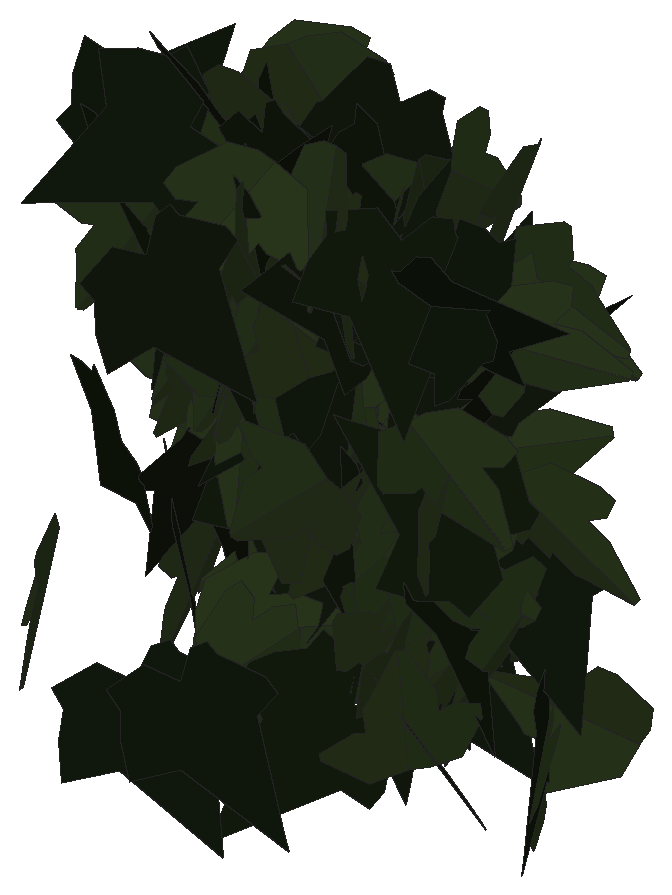
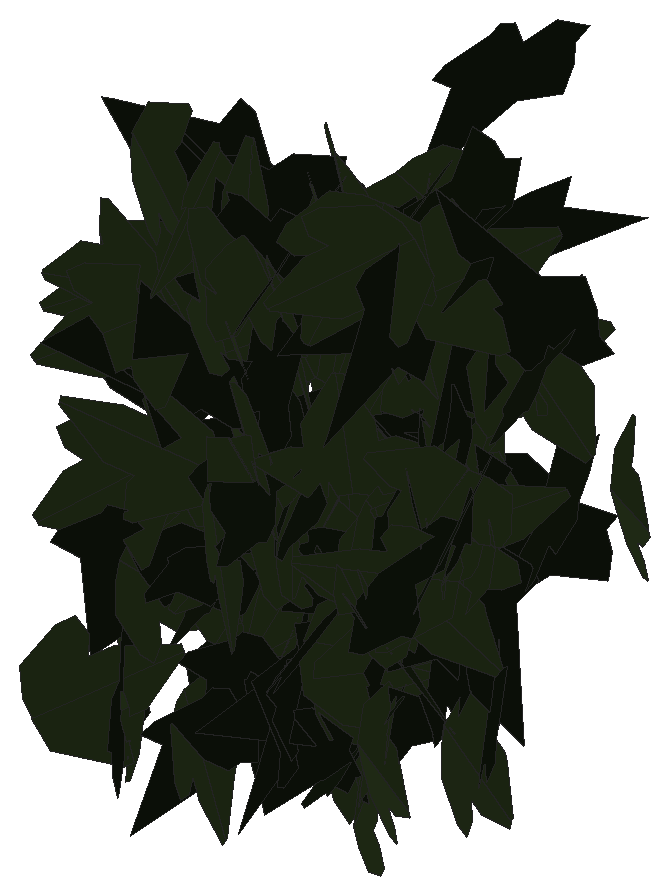
# SketchUp Ruby script. Lengths in inches.
U = 1.inch
M = Sketchup.active_model
def pt(a) = Geom::Point3d.new(a.map { |v| v * U })
def face(e, loops, mat)
  f = e.add_face(loops[0].map { |a| pt(a) })
  loops[1..].each { |l| e.add_face(l.map { |a| pt(a) }).erase! }
  f.material = f.back_material = mat if mat
  f
end
# faces: each face lists its corners as indices into pts; further lists are holes
def faces(e, pts, list, mat = nil) = list.each { |f| face(e, (f[0].is_a?(Array) ? f : [f]).map { |l| l.map { |i| pts[i] } }, mat) }
# xy, xz, yz: faces in a plane at the given z, y or x. An outline is a flat list of corners, or four numbers for a rectangle; further outlines are holes
def ring(l) = l.size == 4 ? [[l[0], l[1]], [l[2], l[1]], [l[2], l[3]], [l[0], l[3]]] : l.each_slice(2).to_a
def flat(e, list, mat, &to3) = list.each { |f| face(e, (f[0].is_a?(Array) ? f : [f]).map { |l| ring(l).map { |u, v| to3.(u, v) } }, mat) }
def xy(e, z, list, mat = nil) = flat(e, list, mat) { |x, y| [x, y, z] }
def xz(e, y, list, mat = nil) = flat(e, list, mat) { |x, z| [x, y, z] }
def yz(e, x, list, mat = nil) = flat(e, list, mat) { |y, z| [x, y, z] }
def lines(e, pts, list) = list.each { |a, b| e.add_line(pt(pts[a]), pt(pts[b])) }
# prism: a flat outline (further loops are holes) pulled along v
def prism(e, loops, v, mat = nil)
  f = face(e, loops, mat); d = Geom::Vector3d.new(v.map { |x| x * U })
  f.pushpull(f.normal.samedirection?(d) ? d.length : -d.length)
end
def box(e, o, s, mat = nil) = prism(e, [[o, [o[0] + s[0], o[1], o[2]], [o[0] + s[0], o[1] + s[1], o[2]], [o[0], o[1] + s[1], o[2]]]], [0, 0, s[2]], mat)
def at(x, y, z, deg = 0) = Geom::Transformation.translation(pt([x, y, z])) * Geom::Transformation.rotation(ORIGIN, Z_AXIS, deg.degrees)
def axes(o, x, y, z) = Geom::Transformation.new([*x, 0, *y, 0, *z, 0, *pt(o).to_a, 1])
def part(name) = M.definitions.add(name)
# library, detail: a bought-in or finely detailed component or shape, given as its bounding box
def library(name, o, s) = part(name).tap { |d| box(d.entities, o, s) }
def detail(e, o, s) = box(e.add_group.entities, o, s)
def put(e, d, t, mat = nil) = e.add_instance(d, t).tap { |i| i.material = mat if mat }
def group(e, t, mat = nil) = e.add_group.tap { |g| g.transformation = t; g.material = mat if mat }.entities
root = M.entities
M.materials.add("efeu1").color = [18, 25, 13]
M.materials.add("efeu2").color = [43, 57, 29]
c1 = part("ivyleaf_9")
p = [[1.54,2.16,1.25],[1.36,2.04,1.19],[-0.21,0.99,0.68],[-0.71,1.11,0.82],[-0.85,0.86,0.67],[-0.8,0.17,0.21],
  [-0.9,-0.01,0.1],[-0.67,-0.16,-0.02],[-0.08,-0.08,-0.05],[-0.03,-0.6,-0.4],[0.65,-0.88,-0.66],[0.83,-0.6,-0.49],
  [1.29,-0.42,-0.43],[1.8125,-0.07,-0.26],[1.21,0.44,0.15]]
faces(c1.entities,p,[[0,1,2,3,4,5,6,7,8,9,10,11,12,13,14]],"efeu1")
c2 = part("ivyleaf_10")
p = [[0,0.5,-0.03],[-0.0625,2.02,-0.43],[-0.19,2.01,-0.46],[-0.54,1.05,-0.29],[-0.52,0.625,-0.18],[-0.83,0.76,-0.28],
  [-1.16,0.64,-0.33],[-1.15,0.33,-0.24],[-0.77,-0.39,0.02],[-0.3,-0.51,0.16],[0.04,-0.48,0.23],[-0.02,2.01,-0.4375],
  [-0.06,2.01,-0.43],[0.04,-0.49,0.23],[0.67,-0.49,0.14],[1.38,0.36,-0.2],[1.375,0.51,-0.24],[0.81,0.65,-0.19],
  [0.62,0.59,-0.15],[0.6,1.09,-0.28],[0.5,1.23,-0.31]]
faces(c2.entities,p,[[0,1,2,3,4,5,6,7,8,9,10],[11,12,0,13,14,15,16,17,18,19,20]],"efeu2")
put(root,c1,axes([25.09,221.01,203.53],[-0.11871,-0.16014,-0.45854],[0.30524,0.34258,-0.19866],[0.37781,-0.3271,0.01643]))
put(root,c1,axes([24.82,220.95,207.18],[0.10215,-0.30245,-0.38482],[-0.06178,0.382,-0.31664],[0.48554,0.11224,0.04067]))
put(root,c2,axes([23.45,221.38,203.92],[0.22421,-0.24414,0.37433],[0.2503,-0.27835,-0.33146],[0.37024,0.33603,-0.00261]))
put(root,c1,axes([24.51,221.16,203.27],[-0.08076,-0.31177,-0.38246],[0.13193,0.3598,-0.32115],[0.47547,-0.15279,0.02415]))
put(root,c2,axes([25.3,222.3,204.79],[-0.31235,-0.09807,0.37792],[-0.36167,-0.10966,-0.32737],[0.1471,-0.47787,-0.00243]))
put(root,c1,axes([23.13,222.6875,204.26],[-0.04041,-0.19305,0.45945],[0.09948,-0.45481,-0.18235],[0.48833,0.07668,0.07517]))
put(root,c2,axes([26.06,222.53,202.68],[-0.29995,-0.38999,-0.08908],[-0.05303,-0.0716,0.492],[-0.39651,0.3046,0.0016]))
put(root,c1,axes([25.28,222.76,202.65],[-0.41912,-0.25084,0.10684],[-0.0888,-0.05966,-0.48842],[0.25778,-0.42839,0.00547]))
put(root,c2,axes([24.54,222.3125,206.63],[0.13243,-0.34063,-0.34123],[-0.03433,0.3463,-0.35902],[0.48092,0.11852,0.06833]))
put(root,c2,axes([24.39,222.71,206.89],[0.33704,0.20832,-0.30497],[-0.25872,-0.16146,-0.39622],[-0.26356,0.42489,-0.00104]))
put(root,c2,axes([24.45,222.34,202.89],[0.07442,0.06049,-0.49072],[0.20924,0.44577,0.08668],[0.44798,-0.21825,0.04103]))
put(root,c1,axes([23.41,223.1,206.89],[-0.2597,-0.24329,0.35123],[-0.23296,-0.26393,-0.35507],[0.35817,-0.34807,0.02373]))
put(root,c2,axes([26.12,222.72,205.27],[-0.41391,-0.09442,-0.26414],[0.26559,0.01954,-0.42318],[0.09023,-0.49062,0.03398]))
put(root,c2,axes([24.7,222.98,205.4],[-0.25897,-0.39411,-0.16617],[-0.09187,-0.13846,0.47158],[-0.41772,0.27478,-0.0007]))
put(root,c2,axes([24.28,222.53,203.11],[0.0175,-0.10886,-0.48769],[0.3533,0.34779,-0.06495],[0.35337,-0.34233,0.08909]))
put(root,c1,axes([25.63,222.97,206.69],[-0.23129,-0.38456,-0.22049],[0.13615,0.17505,-0.44813],[0.42186,-0.26734,0.02374]))
put(root,c1,axes([25.77,223.12,202.33],[0.41797,-0.23769,-0.13714],[0.12911,-0.05017,0.48043],[-0.24215,-0.43702,0.01944]))
put(root,c1,axes([26.53,222.81,206.5],[-0.39364,0.24285,0.18993],[-0.16097,0.10081,-0.46252],[-0.26294,-0.42528,-0.00119]))
put(root,c2,axes([24.89,223.15,206.22],[0.09897,-0.12912,-0.47279],[0.2886,-0.37449,0.16269],[-0.39613,-0.30509,0.0004]))
put(root,c2,axes([24.84,223.03,206.99],[0.41456,-0.23626,0.14941],[0.12797,-0.07721,-0.47714],[0.24853,0.43384,-0.00355]))
put(root,c2,axes([25.7,223.17,204.35],[0.15333,-0.28761,-0.37917],[0.21672,-0.31246,0.32465],[-0.4237,-0.26391,0.02884]))
put(root,c2,axes([23.08,223.11,206.07],[-0.22091,-0.3648,0.26099],[-0.13727,-0.22198,-0.42647],[0.42703,-0.26008,-0.00208]))
put(root,c1,axes([26,222.94,206.3125],[0.36254,0.1201,-0.32271],[0.30144,0.11581,0.38174],[0.16644,-0.47134,0.01156]))
put(root,c2,axes([24,223.05,204.8125],[0.46185,-0.13751,0.13336],[0.12745,-0.03927,-0.48189],[0.14301,0.47911,-0.00122]))
put(root,c1,axes([24.85,223.39,205.89],[0.16987,-0.39314,-0.25804],[0.12876,-0.22499,0.42755],[-0.45229,-0.21171,0.0248]))
put(root,c2,axes([24.07,223.25,205.34],[-0.18716,-0.39384,0.24466],[-0.10329,-0.2218,-0.43605],[0.452,-0.21376,0.00166]))
put(root,c2,axes([24.03,223.42,204.92],[-0.14466,-0.11216,-0.46529],[-0.25801,-0.39113,0.1745],[-0.40312,0.29058,0.05528]))
put(root,c2,axes([25.49,223.05,202.8],[0.04223,-0.46361,0.18244],[-0.02567,0.18082,0.46545],[-0.49755,-0.04868,-0.00853]))
put(root,c2,axes([23.4,223.43,204.66],[-0.04705,-0.38464,-0.31597],[-0.05126,-0.31195,0.38738],[-0.49514,0.06884,-0.01008]))
put(root,c1,axes([22.64,223.37,206.23],[0.21714,-0.41322,0.17917],[0.07533,-0.16279,-0.46672],[0.44404,0.22968,-0.00844]))
put(root,c1,axes([23.43,223.41,205.37],[0.19939,-0.42948,0.16059],[0.08327,-0.13829,-0.47323],[0.4509,0.21546,0.01637]))
put(root,c2,axes([24.81,223.17,203.59],[-0.24735,-0.41011,0.14364],[0.07314,0.12363,0.47892],[-0.42833,0.25793,-0.00117]))
put(root,c1,axes([23.3125,223.3,207.16],[0.35031,-0.26954,0.23373],[0.18412,-0.14398,-0.442],[0.30558,0.39575,-0.00162]))
put(root,c2,axes([23.81,223.48,204.44],[0.24613,-0.2155,0.37813],[0.275,-0.2597,-0.32701],[0.33733,0.36894,-0.00932]))
put(root,c1,axes([24.5,223.33,205.2],[-0.48369,0.10719,-0.06748],[0.06572,-0.01534,-0.49542],[-0.10828,-0.48813,0.00075]))
put(root,c1,axes([23.5,223.5,203.11],[-0.01921,-0.02785,0.49885],[0.16196,-0.47261,-0.02015],[0.47265,0.16082,0.02718]))
put(root,c2,axes([25.37,223.15,203],[-0.17631,-0.4115,0.22267],[0.0885,0.20433,0.44768],[-0.45944,0.19728,0.00079]))
put(root,c1,axes([26.13,223.36,204.2],[-0.35162,-0.30457,-0.1833],[-0.12288,-0.1378,0.46466],[-0.33356,0.37182,0.02206]))
put(root,c1,axes([25.65,223.48,203.46],[0.20862,-0.41565,0.1836],[0.08121,-0.16467,-0.46507],[0.44708,0.22387,-0.0012]))
put(root,c1,axes([23.55,223.41,205.66],[-0.01234,-0.11139,0.48728],[0.37782,-0.3212,-0.06386],[0.32726,0.36663,0.0921]))
put(root,c2,axes([25.3,223.55,205.63],[-0.08073,-0.06027,-0.48974],[-0.38391,-0.3041,0.10071],[-0.31,0.39229,0.00283]))
put(root,c1,axes([24.06,223.3,206.93],[0.29093,-0.38934,-0.11738],[-0.05731,0.10363,-0.48577],[0.40259,0.2961,0.01567]))
put(root,c1,axes([24.36,223.4,204.21],[-0.16407,-0.07082,-0.46698],[0.45244,0.11835,-0.17691],[0.13559,-0.4806,0.02525]))
put(root,c2,axes([25.06,223.49,202.83],[-0.20784,0.34887,0.29171],[0.14079,-0.25561,0.40601],[0.43241,0.2509,0.00801]))
put(root,c1,axes([23.03,223.6,202.84],[-0.07724,0.03653,0.49265],[0.05676,-0.49467,0.04558],[0.49073,0.06296,0.07227]))
put(root,c2,axes([23.52,223.3,205.86],[-0.43206,-0.2515,-0.00859],[0.00819,0.00301,-0.49992],[0.25151,-0.43213,0.00152]))
put(root,c1,axes([22.73,223.27,206.4],[-0.228,0.12218,0.42789],[0.38883,-0.17911,0.25833],[0.2164,0.45055,-0.01334]))
put(root,c2,axes([25.54,223.14,203.83],[-0.21703,-0.27002,-0.36054],[0.24348,0.26638,-0.34607],[0.37897,-0.32578,0.01587]))
put(root,c1,axes([23.53,223.38,204.1],[-0.05705,0.39622,-0.2996],[0.04833,-0.29571,-0.40028],[-0.49438,-0.07462,-0.00456]))
put(root,c1,axes([24.24,223.4,205.25],[-0.2427,-0.23885,-0.36613],[0.25083,0.26688,-0.34038],[0.35802,-0.34889,-0.00972]))
put(root,c2,axes([23.27,223.73,205.04],[-0.00219,-0.17029,0.4701],[0.15558,-0.447,-0.16119],[0.47517,0.14557,0.05495]))
put(root,c1,axes([25.4,223.22,205.75],[-0.38232,-0.02449,0.32129],[0.32122,0.01031,0.38303],[-0.02538,0.49929,0.00785]))
put(root,c1,axes([23.61,223.43,205.21],[-0.22258,-0.22322,-0.38811],[0.31807,0.2262,-0.31251],[0.3151,-0.38601,0.0413]))
put(root,c2,axes([23.46,223.5625,204.53],[0.15313,0.183,0.43939],[-0.28938,-0.33067,0.23857],[0.3779,-0.32737,0.00464]))
put(root,c2,axes([23.47,223.61,206.74],[-0.23311,-0.02963,-0.44134],[-0.40345,-0.19029,0.22587],[-0.18135,0.46142,0.06481]))
put(root,c1,axes([23.52,223.56,204.71],[0.00005,0.28885,0.40812],[-0.03866,-0.4069,0.28799],[0.4985,-0.03159,0.02229]))
put(root,c2,axes([23.8125,223.59,206.51],[0.10745,-0.46729,0.14177],[0.02984,-0.13861,-0.47948],[0.48741,0.1115,-0.0019]))
put(root,c1,axes([24.16,223.75,202.54],[0.07627,-0.4068,0.28053],[0.10945,-0.2629,-0.41098],[0.48187,0.1241,0.04895]))
put(root,c2,axes([24.19,223.26,205.01],[-0.17669,-0.37353,-0.28152],[0.13197,0.2489,-0.41308],[0.44874,-0.22028,0.01063]))
put(root,c2,axes([25.79,223.23,203.83],[-0.23393,-0.20855,-0.38959],[0.29568,0.25373,-0.31336],[0.3284,-0.377,0.00462]))
put(root,c2,axes([23.21,223.72,204.49],[-0.22901,0.14281,0.4209],[0.25674,-0.344,0.25641],[0.36282,0.33357,0.08424]))
put(root,c2,axes([23.03,223.68,204.75],[-0.05843,0.07951,-0.49017],[0.31615,-0.37465,-0.09845],[-0.38293,-0.32143,-0.00649]))
put(root,c2,axes([24.89,223.28,203.85],[-0.24423,-0.3262,-0.28974],[0.18152,0.22597,-0.40742],[0.39674,-0.30419,0.00804]))
put(root,c2,axes([23.76,223.5,204.47],[0.04126,-0.4981,-0.01376],[-0.00084,0.01374,-0.49981],[0.49829,0.04127,0.00029]))
put(root,c2,axes([24.4,223.21,206.31],[-0.00525,-0.32404,-0.38075],[0.01671,0.38045,-0.32401],[0.49969,-0.01613,0.00684]))
put(root,c2,axes([24.05,223.79,202],[0.04833,-0.03837,0.49618],[0.35389,-0.34784,-0.06137],[0.34989,0.35712,-0.00646]))
put(root,c2,axes([24.18,223.84,203.08],[-0.02287,0.06723,0.49493],[-0.11417,-0.48304,0.06034],[0.48625,-0.11025,0.03744]))
put(root,c2,axes([23.12,223.76,202.91],[0.12453,-0.40463,0.26602],[0.09025,-0.25046,-0.42323],[0.47576,0.15343,0.01066]))
put(root,c1,axes([24.1,223.67,203.96],[-0.20609,-0.40831,-0.20201],[0.11622,0.16726,-0.45664],[0.44048,-0.23517,0.02596]))
put(root,c2,axes([24.25,223.89,203.43],[-0.03531,-0.16331,0.47126],[-0.11283,-0.45757,-0.16702],[0.48582,-0.11814,-0.00454]))
put(root,c2,axes([26.13,223.88,203.41],[0.04509,-0.32795,0.37472],[0.04467,-0.37207,-0.33101],[0.49595,0.06333,-0.00425]))
put(root,c2,axes([24.13,223.76,202.33],[-0.24723,-0.00181,0.4346],[0.40742,-0.17501,0.23104],[0.15128,0.46837,0.08801]))
put(root,c1,axes([24.07,223.16,206.39],[0.1822,0.26365,0.38379],[0.19284,0.33239,-0.31989],[-0.42381,0.26459,0.01944]))
put(root,c1,axes([24.65,223.77,204.15],[-0.40592,-0.23839,-0.16852],[0.14529,0.08538,-0.47075],[0.25322,-0.43114,-0.00004]))
put(root,c1,axes([24.77,223.96,206.57],[0.03506,-0.4205,0.26823],[0.00707,-0.26845,-0.42177],[0.49872,0.03337,-0.01288]))
put(root,c1,axes([23.12,223.78,205.34],[0.04158,0.00481,-0.49824],[0.49697,-0.03643,0.04113],[-0.03591,-0.49865,-0.00781]))
put(root,c2,axes([23.75,223.91,204.7],[0.01763,-0.42777,0.25827],[0.01357,-0.25793,-0.42812],[0.4995,0.02211,0.00251]))
put(root,c2,axes([25.17,223.9375,206.43],[-0.05088,-0.4056,-0.28793],[0.04867,-0.2921,0.40287],[-0.49502,0.01297,0.06921]))
put(root,c2,axes([26.19,223.49,205.88],[-0.15613,-0.09598,-0.4652],[0.42308,0.1945,-0.18212],[0.21593,-0.45051,0.02048]))
put(root,c2,axes([26.06,223.9,207.09],[0.17997,-0.42651,0.18894],[0.06653,-0.17697,-0.46288],[0.46172,0.19175,-0.00695]))
put(root,c2,axes([25.39,223.89,206.24],[0.30073,-0.37521,0.13704],[0.08397,-0.10832,-0.48085],[0.39053,0.31222,-0.00214]))
put(root,c2,axes([24.47,224.1,204.39],[-0.00988,-0.13182,0.48221],[0.22931,-0.42976,-0.11278],[0.4442,0.21892,0.06895]))
put(root,c2,axes([26.54,223.49,201.97],[0.1925,-0.15064,0.43618],[-0.31392,0.30365,0.24342],[-0.33823,-0.36757,0.02233]))
put(root,c1,axes([26.22,224.05,202.51],[-0.07074,0.02059,-0.49454],[0.43633,-0.23328,-0.07213],[-0.2337,-0.44177,0.01504]))
put(root,c2,axes([25.43,223.9,205.73],[0.25399,-0.39764,-0.16545],[0.08733,-0.14054,0.47183],[-0.42174,-0.26857,-0.00194]))
put(root,c2,axes([23.53,223.99,204.29],[-0.2417,-0.22638,0.37461],[-0.25408,-0.27589,-0.33065],[0.35641,-0.3502,0.01833]))
put(root,c2,axes([24.95,223.94,206.56],[-0.26012,-0.37863,0.19742],[-0.10007,-0.17068,-0.45919],[0.41512,-0.2784,0.01302]))
put(root,c2,axes([24.48,224.05,204.51],[-0.17612,-0.35816,0.30117],[-0.10224,-0.28456,-0.39821],[0.45665,-0.20185,0.02699]))
put(root,c1,axes([26,223.46,205.32],[-0.06951,0.40079,-0.29075],[-0.04801,0.28676,0.40677],[0.49281,0.08446,-0.00138]))
put(root,c1,axes([24.65,223.97,202.74],[-0.2823,-0.17944,-0.37163],[0.33014,0.17196,-0.33382],[0.24761,-0.43385,0.02139]))
put(root,c1,axes([24.8125,223.56,202.57],[-0.01535,-0.04377,0.49784],[0.11771,0.48375,0.04616],[-0.48571,0.11861,-0.00455]))
put(root,c2,axes([23.72,223.97,204.59],[-0.13665,-0.47684,0.06288],[-0.0071,-0.06336,-0.49592],[0.48091,-0.13643,0.01055]))
put(root,c1,axes([24.07,223.67,203.07],[0.09582,0.01646,-0.49046],[0.23477,0.43729,0.06054],[0.43093,-0.24189,0.07608]))
put(root,c1,axes([24.56,223.66,203.11],[0.13395,-0.18121,-0.44634],[-0.26586,0.35852,-0.22534],[0.40172,0.2977,-0.0003]))
put(root,c2,axes([23.67,224.16,202.8],[0.24074,-0.30507,0.31461],[0.18053,-0.25804,-0.38836],[0.39932,0.30058,-0.01409]))
put(root,c1,axes([24.17,223.92,204.1],[-0.42411,0.26456,0.01166],[-0.00989,0.00617,-0.49986],[-0.26464,-0.42423,0]))
put(root,c1,axes([26.05,223.9375,203.77],[-0.19437,-0.28199,-0.36428],[0.20084,0.30396,-0.34245],[0.41459,-0.27945,-0.00489]))
put(root,c2,axes([24.74,223.95,206.4],[0.32568,-0.37089,-0.07984],[-0.05282,0.05988,-0.49358],[0.37569,0.32994,-0.00018]))
put(root,c2,axes([24.16,224.01,204.71],[0.39894,-0.02416,0.30044],[0.29967,-0.02161,-0.39966],[0.0323,0.49895,-0.00276]))
put(root,c2,axes([26.25,223.91,204.27],[-0.33167,0.04926,-0.3709],[0.36879,-0.04066,-0.33518],[-0.06318,-0.4959,-0.00936]))
put(root,c1,axes([25.16,224.18,204.125],[-0.12341,-0.48295,-0.03911],[0.0052,0.03904,-0.49845],[0.4845,-0.12344,-0.00461]))
put(root,c1,axes([24.76,223.96,203.13],[-0.13216,-0.29264,-0.38327],[0.21035,0.32261,-0.31886],[0.43392,-0.24552,0.03784]))
put(root,c1,axes([24.63,224.13,204.57],[0.27502,-0.38023,0.17258],[-0.09568,0.14378,0.46923],[-0.40646,-0.29112,0.00633]))
put(root,c1,axes([24.68,224.11,207.06],[-0.422,-0.14548,-0.22529],[0.20774,0.08829,-0.44615],[0.16959,-0.47015,-0.01407]))
put(root,c1,axes([25.63,223.83,205.06],[-0.39212,0.00661,0.31016],[0.31015,-0.00334,0.39217],[0.00725,0.49995,-0.00148]))
put(root,c1,axes([22.85,224.38,204.91],[-0.00962,-0.27002,0.42071],[0.00685,-0.42082,-0.26993],[0.49986,0.00057,0.0118]))
put(root,c2,axes([25.59,223.74,206.97],[0.0908,-0.30672,-0.38429],[0.07421,0.39486,-0.29762],[0.48605,-0.00299,0.11723]))
put(root,c2,axes([25.74,223.93,204.58],[0.13252,0.01766,-0.4818],[0.48014,0.04035,0.13354],[0.0436,-0.49806,-0.00626]))
put(root,c2,axes([26.64,224.23,202.28],[-0.20406,-0.07659,-0.44999],[-0.41914,-0.16376,0.21795],[-0.18077,0.46617,0.00263]))
put(root,c2,axes([23.04,223.95,205.29],[0.37033,0.21599,0.25731],[0.2073,0.15443,-0.42799],[-0.26435,0.42368,0.02483]))
put(root,c2,axes([23.88,223.99,207.23],[-0.42527,-0.18654,-0.18535],[0.17428,0.06398,-0.46426],[0.19692,-0.45947,0.0106]))
put(root,c2,axes([26,224.08,206.0625],[0.10947,0.03278,0.48677],[0.47975,0.08341,-0.1135],[-0.08864,0.4919,-0.01319]))
put(root,c2,axes([25.36,224.2,202.54],[0.08228,-0.49125,0.04368],[0.00714,-0.04309,-0.49809],[0.49313,0.08259,-0.00007]))
put(root,c2,axes([24.875,224.16,204.95],[0.45795,-0.06033,-0.19142],[-0.18983,0.02462,-0.46191],[0.06516,0.49574,-0.00036]))
put(root,c2,axes([25.23,224.1,204.31],[0.15821,-0.45784,-0.12391],[-0.03756,0.11812,-0.48439],[0.47282,0.16258,0.00298]))
put(root,c1,axes([23.62,223.79,206.78],[0.03344,-0.02508,-0.49825],[-0.30867,0.39126,-0.04041],[0.39192,0.3103,0.01068]))
put(root,c1,axes([24.54,224.31,204.9],[0.27268,-0.32246,0.2677],[0.18216,-0.19644,-0.42217],[0.37744,0.32777,0.01035]))
put(root,c2,axes([24.97,224.1,205.32],[0.30574,-0.34601,-0.19183],[-0.12818,0.14273,-0.46173],[0.37429,0.33152,-0.00143]))
put(root,c2,axes([23.7,224.02,207.12],[-0.2633,-0.09296,-0.41476],[0.39923,0.11338,-0.27886],[0.14589,-0.47802,0.01452]))
put(root,c1,axes([23.23,224.27,204.54],[0.27566,-0.22995,0.34804],[0.29207,-0.19146,-0.35783],[0.29784,0.40058,0.02876]))
put(root,c2,axes([23.99,224.05,205.125],[0.41224,0.27566,-0.06379],[0.04891,0.0416,0.49586],[0.27869,-0.41507,0.00733]))
put(root,c1,axes([24.77,224.14,205.49],[0.15337,-0.29696,0.37188],[-0.12713,0.35094,0.33268],[-0.4586,-0.1966,0.03214]))
put(root,c1,axes([25.06,224.09,202.67],[0.05322,-0.32687,-0.3746],[0.03568,0.37828,-0.32501],[0.49588,0.00786,0.06359]))
put(root,c2,axes([25.93,224.13,205.85],[-0.28179,-0.03152,-0.41183],[0.40951,0.04364,-0.28354],[0.05382,-0.49709,0.00122]))
put(root,c1,axes([23.95,224.32,204.03],[0.21982,-0.44225,-0.07807],[-0.03503,0.06977,-0.49387],[0.44772,0.2226,-0.00031]))
put(root,c2,axes([23.29,224.01,204.41],[0.10963,-0.01696,-0.48754],[0.43376,0.23205,0.08947],[0.22323,-0.44257,0.06559]))
